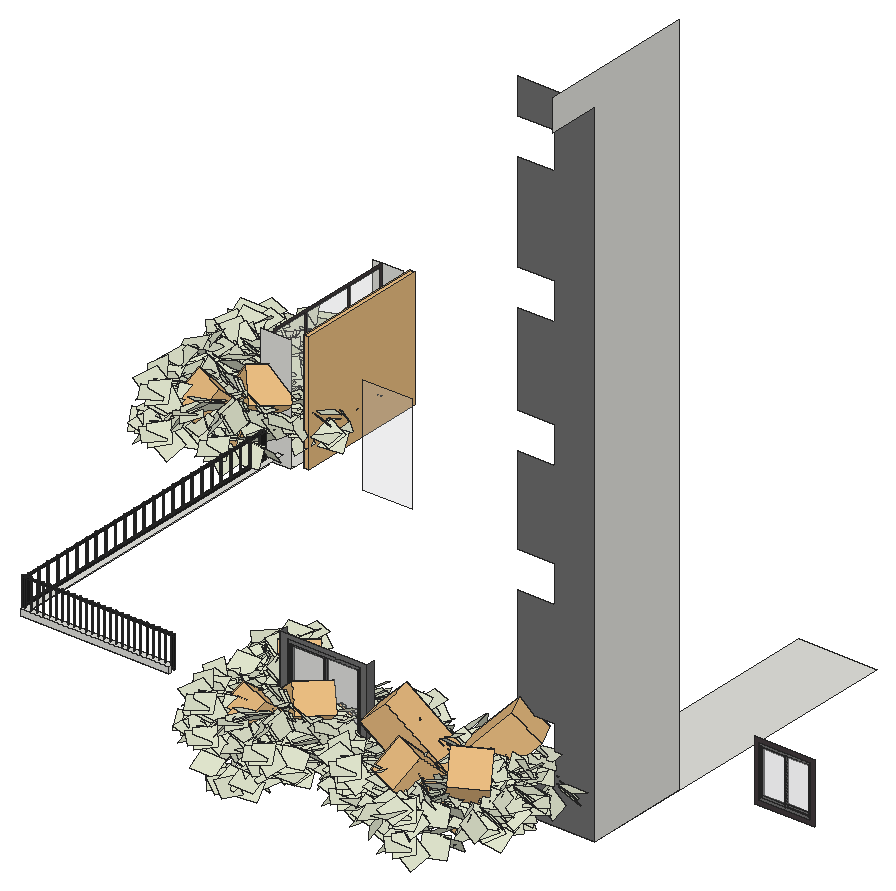
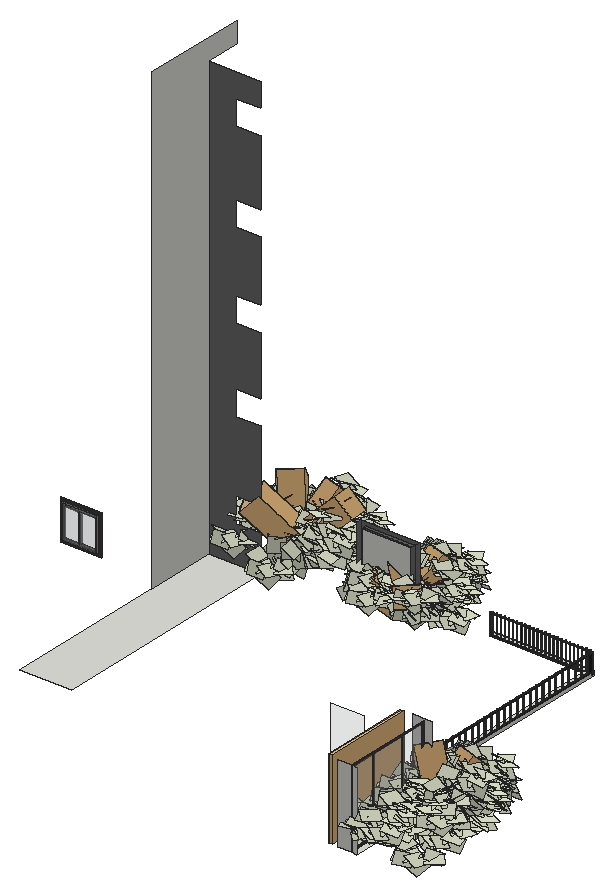
# SketchUp Ruby script. Lengths in inches.
U = 1.inch
M = Sketchup.active_model
def pt(a) = Geom::Point3d.new(a.map { |v| v * U })
def face(e, loops, mat)
  f = e.add_face(loops[0].map { |a| pt(a) })
  loops[1..].each { |l| e.add_face(l.map { |a| pt(a) }).erase! }
  f.material = f.back_material = mat if mat
  f
end
# faces: each face lists its corners as indices into pts; further lists are holes
def faces(e, pts, list, mat = nil) = list.each { |f| face(e, (f[0].is_a?(Array) ? f : [f]).map { |l| l.map { |i| pts[i] } }, mat) }
# xy, xz, yz: faces in a plane at the given z, y or x. An outline is a flat list of corners, or four numbers for a rectangle; further outlines are holes
def ring(l) = l.size == 4 ? [[l[0], l[1]], [l[2], l[1]], [l[2], l[3]], [l[0], l[3]]] : l.each_slice(2).to_a
def flat(e, list, mat, &to3) = list.each { |f| face(e, (f[0].is_a?(Array) ? f : [f]).map { |l| ring(l).map { |u, v| to3.(u, v) } }, mat) }
def xy(e, z, list, mat = nil) = flat(e, list, mat) { |x, y| [x, y, z] }
def xz(e, y, list, mat = nil) = flat(e, list, mat) { |x, z| [x, y, z] }
def yz(e, x, list, mat = nil) = flat(e, list, mat) { |y, z| [x, y, z] }
def lines(e, pts, list) = list.each { |a, b| e.add_line(pt(pts[a]), pt(pts[b])) }
# prism: a flat outline (further loops are holes) pulled along v
def prism(e, loops, v, mat = nil)
  f = face(e, loops, mat); d = Geom::Vector3d.new(v.map { |x| x * U })
  f.pushpull(f.normal.samedirection?(d) ? d.length : -d.length)
end
def box(e, o, s, mat = nil) = prism(e, [[o, [o[0] + s[0], o[1], o[2]], [o[0] + s[0], o[1] + s[1], o[2]], [o[0], o[1] + s[1], o[2]]]], [0, 0, s[2]], mat)
def at(x, y, z, deg = 0) = Geom::Transformation.translation(pt([x, y, z])) * Geom::Transformation.rotation(ORIGIN, Z_AXIS, deg.degrees)
def axes(o, x, y, z) = Geom::Transformation.new([*x, 0, *y, 0, *z, 0, *pt(o).to_a, 1])
def part(name) = M.definitions.add(name)
# library, detail: a bought-in or finely detailed component or shape, given as its bounding box
def library(name, o, s) = part(name).tap { |d| box(d.entities, o, s) }
def detail(e, o, s) = box(e.add_group.entities, o, s)
def put(e, d, t, mat = nil) = e.add_instance(d, t).tap { |i| i.material = mat if mat }
def group(e, t, mat = nil) = e.add_group.tap { |g| g.transformation = t; g.material = mat if mat }.entities
root = M.entities
M.materials.add("Celtis_australis_s cópia1").color = [224, 229, 205]
M.materials.add("Niraj_Hair_Dark").color = [109, 109, 109]
M.materials.add("[Asphalt New]").color = [67, 60, 62]
M.materials.add("[Color M08]").color = [30, 30, 30]
M.materials.add("[CoolGray4]").color = [225, 226, 230]
M.materials["[CoolGray4]"].alpha = 0.26
M.materials.add("aubin blanc").color = [238, 236, 240]
M.materials.add("bark_cherry").color = [99, 76, 62]
c1 = part("leaf1\#1")
p = [[1.6,6.78,0.04],[-9.34,-4.04,0.02],[2.67,-16.2,2.05],[13.62,-5.38,2.07]]
faces(c1.entities,p,[[0,1,2,3]],"Celtis_australis_s cópia1")
c2 = part("leaf_group1\#1")
put(c2.entities,c1,axes([-0.06,3.68,7.3125],[0.53029,-0.80282,-0.27253],[0.82812,0.42159,0.36943],[-0.18168,-0.42159,0.8884]))
put(c2.entities,c1,axes([6.4375,-3.58,5.23],[1,0,0],[0,0.98927,0.14608],[0,-0.14608,0.98927]))
put(c2.entities,c1,axes([-0.99,3.68,1.22],[0.57591,-0.80282,0.15431],[0.36532,0.42159,0.82994],[-0.73135,-0.42159,0.53609]))
put(c2.entities,c1,axes([18.71,8.59,4.39],[0.33053,0.77491,0.53877],[-0.79988,-0.073,0.5957],[0.50094,-0.62785,0.5957]))
put(c2.entities,c1,axes([13.16,0.76,0.89],[0.89618,0.3501,0.27256],[-0.44248,0.65988,0.60727],[0.03275,-0.66482,0.74628]))
put(c2.entities,c1,axes([4.53,7.98,7.3125],[-0.1927,0.94265,-0.27253],[0.88368,0.28746,0.36943],[-0.42658,0.16964,0.8884]))
put(c2.entities,c1,axes([12.46,21.28,7.16],[0.85019,0.38493,0.35918],[0.30538,-0.91629,0.25914],[-0.42887,0.11063,0.89657]))
put(c2.entities,c1,axes([6.53,15.18,2.59],[0.70711,0.70711,0],[0.5,-0.5,0.70711],[-0.5,0.5,0.70711]))
put(c2.entities,c1,axes([-3.17,8.15,3.46],[-0.03719,0.74973,0.66069],[0.94096,-0.19634,0.27576],[-0.33647,-0.63194,0.69817]))
put(c2.entities,c1,axes([23.03,17.79,4.39],[0.78166,-0.31422,0.53877],[-0.61722,-0.51398,0.5957],[-0.08973,0.79818,0.5957]))
put(c2.entities,c1,axes([14.78,21.52,3.21],[0.67246,-0.04394,0.73882],[-0.28657,-0.93583,0.20517],[-0.6824,0.3497,0.64191]))
put(c2.entities,c1,axes([10.37,-1.8125,9],[0.99279,-0.06448,-0.101],[0.11527,0.74421,0.65792],[0.03275,-0.66482,0.74628]))
put(c2.entities,c1,axes([1.45,16.1875,2.9375],[-0.2106,-0.86579,-0.45394],[0.96054,-0.26957,0.06852],[-0.18168,-0.42159,0.8884]))
c3 = library("branch1\#2",[0,0,0],[33.4,33.29,108.01])
c4 = library("fronceur+aubin+blanc+(3)",[-47.99,-0.29,1.66],[95.37,4.84,114.09])
c5 = part("branch2\#1")
p = [[13.74,0.36,0.5],[11.5,11.3125,10.98],[14.125,0.95,0],[14.97,0.95,0.19],[12.12,10.6875,11.67],[15.1,0.36,0.82],
  [11.05,10.4375,11.49],[14.34,0,1.01],[6.08,18.54,23.51],[6.83,18.32,23.89],[6.09,17.93,24.13],[3.27,29.37,34],
  [3.27,29.68,33.56],[3.73,29.59,33.82],[0,43.16,40.74],[0,43.16,40.75],[0.01,43.16,40.75],[5.59,23.2,32.77],
  [4.65,30.48,39.08],[1.92,39.79,43.02],[5.09,28.47,41.41]]
faces(c5.entities,p,[[0,1,2],[2,1,3],[3,4,5],[3,1,4],[6,0,7],[0,6,1],[5,6,7],[6,5,4],
  [6,8,1],[1,9,4],[9,1,8],[8,6,10],[4,10,6],[10,4,9],[10,11,8],[8,12,9],
  [12,8,11],[10,9,11],[13,11,9],[13,9,12],[14,12,11,15],[12,14,16,13],[13,16,15,11]],"bark_cherry")
lines(c5.entities,p,[[17,18],[11,19],[20,17],[17,10]])
c6 = part("Window sash")
g1 = group(c6.entities,at(0.98,0,0),"Niraj_Hair_Dark")
prism(g1,[[[-0.98,0,0],[30.98,0,0],[30.98,0,45.6],[-0.98,0,45.6]],[[29.01,0,43.625],[29.01,0,1.97],[0.98,0,1.97],[0.98,0,43.625]]],[0,1.18,0])
g2 = group(c6.entities,at(1.97,0.59,1.97))
xz(g2,0,[[0,0,28.03,41.66]],"[CoolGray4]")
c7 = part("Twin sash window")
put(c7.entities,c6,at(31.97,2.82,1.97))
put(c7.entities,c6,at(1.97,1.25,1.97))
g3 = group(c7.entities,at(0,0,0),"Niraj_Hair_Dark")
prism(g3,[[[65.9,4.72,0],[0,4.72,0],[0,4.72,49.53],[65.9,4.72,49.53]],[[1.97,4.72,47.5625],[1.97,4.72,1.97],[63.93,4.72,1.97],[63.93,4.72,47.5625]]],[0,-4.72,0])
c8 = part("Group\#428")
prism(c8.entities,[[[0,1.97,0],[0,1.97,1.18],[0,0,1.18],[0,0,0]],[[0,1.92,1.13],[0,1.92,0.05],[0,0.05,0.05],[0,0.05,1.13]]],[98.43,0,0])
c9 = part("Group\#430")
xy(c9.entities,0,[[0.3,0,0.22,0.01,0.15,0.04,0.09,0.09,0.04,0.15,0.01,0.22,0,0.3,0.3,0.3],[0.3,0,0.3,0.3,0.59,0.3,0.58,0.22,0.55,0.15,0.5,0.09,0.44,0.04,0.37,0.01],[0,0.3,0.01,0.37,0.04,0.44,0.09,0.5,0.15,0.55,0.22,0.58,0.3,0.59,0.3,0.3],[0.3,0.3,0.3,0.59,0.37,0.58,0.44,0.55,0.5,0.5,0.55,0.44,0.58,0.37,0.59,0.3]])
xy(c9.entities,39.37,[[0.3,0,0.37,0.01,0.44,0.04,0.5,0.09,0.55,0.15,0.58,0.22,0.59,0.3,0.58,0.37,0.55,0.44,0.5,0.5,0.44,0.55,0.37,0.58,0.3,0.59,0.22,0.58,0.15,0.55,0.09,0.5,0.04,0.44,0.01,0.37,0,0.3,0.01,0.22,0.04,0.15,0.09,0.09,0.15,0.04,0.22,0.01]])
p = [[0.09,0.09,0],[0.15,0.04,0],[0.15,0.04,39.37],[0.09,0.09,39.37],[0.22,0.01,0],[0.22,0.01,39.37],
  [0.3,0,0],[0.3,0,39.37],[0.37,0.01,0],[0.37,0.01,39.37],[0.44,0.04,0],[0.44,0.04,39.37],
  [0.5,0.09,0],[0.5,0.09,39.37],[0.01,0.22,0],[0.04,0.15,0],[0.04,0.15,39.37],[0.01,0.22,39.37],
  [0.55,0.15,0],[0.55,0.15,39.37],[0.58,0.22,0],[0.58,0.22,39.37],[0,0.3,0],[0,0.3,39.37],
  [0.59,0.3,0],[0.59,0.3,39.37],[0.01,0.37,0],[0.01,0.37,39.37],[0.58,0.37,0],[0.58,0.37,39.37],
  [0.09,0.5,0],[0.04,0.44,0],[0.04,0.44,39.37],[0.09,0.5,39.37],[0.55,0.44,0],[0.5,0.5,0],
  [0.5,0.5,39.37],[0.55,0.44,39.37],[0.15,0.55,0],[0.15,0.55,39.37],[0.44,0.55,0],[0.44,0.55,39.37],
  [0.22,0.58,0],[0.22,0.58,39.37],[0.3,0.59,0],[0.3,0.59,39.37],[0.37,0.58,0],[0.37,0.58,39.37]]
faces(c9.entities,p,[[0,1,2,3],[1,4,5,2],[4,6,7,5],[6,8,9,7],[8,10,11,9],[10,12,13,11],[14,15,16,17],[15,0,3,16],
  [12,18,19,13],[18,20,21,19],[22,14,17,23],[20,24,25,21],[26,22,23,27],[24,28,29,25],[30,31,32,33],[31,26,27,32],
  [34,35,36,37],[28,34,37,29],[38,30,33,39],[35,40,41,36],[42,38,39,43],[44,42,43,45],[46,44,45,47],[40,46,47,41]])
c10 = part("Group\#429")
prism(c10.entities,[[[0.01,0.22,35.83],[0,0.3,35.83],[0.01,0.37,35.83],[0.04,0.44,35.83],[0.09,0.5,35.83],[0.15,0.55,35.83],[0.22,0.58,35.83],[0.3,0.59,35.83],[0.37,0.58,35.83],[0.44,0.55,35.83],[0.5,0.5,35.83],[0.55,0.44,35.83],[0.58,0.37,35.83],[0.59,0.3,35.83],[0.58,0.22,35.83],[0.55,0.15,35.83],[0.5,0.09,35.83],[0.44,0.04,35.83],[0.37,0.01,35.83],[0.3,0,35.83],[0.22,0.01,35.83],[0.15,0.04,35.83],[0.09,0.09,35.83],[0.04,0.15,35.83]]],[0,0,3.54])
c11 = part("Balcony railing panel")
g4 = group(c11.entities,at(0,0,0))
put(g4,c8,axes([0,0,39.76],[1,0,0],[0,0,-1],[0,1,0]),"[Color M08]")
put(g4,c8,axes([0,0,1.97],[1,0,0],[0,0,-1],[0,1,0]),"[Color M08]")
put(g4,c8,axes([98.43,0,37.8],[0,0,-0.364],[-1,0,0],[0,1,0]),"[Color M08]")
put(g4,c8,axes([1.97,0,37.8],[0,0,-0.364],[-1,0,0],[0,1,0]),"[Color M08]")
g5 = group(c11.entities,at(1.67,0.3,1.97))
put(g5,c9,at(78.74,0,0),"[Color M08]")
put(g5,c9,at(90.55,0,0),"[Color M08]")
put(g5,c9,at(82.68,0,0),"[Color M08]")
put(g5,c9,at(86.61,0,0),"[Color M08]")
put(g5,c9,at(66.93,0,0),"[Color M08]")
put(g5,c9,at(11.8125,0,0),"[Color M08]")
put(g5,c9,at(15.75,0,0),"[Color M08]")
put(g5,c9,at(47.24,0,0),"[Color M08]")
put(g5,c9,at(59.06,0,0),"[Color M08]")
put(g5,c10,at(0,0,0),"[Color M08]")
put(g5,c9,at(39.37,0,0),"[Color M08]")
put(g5,c9,at(62.99,0,0),"[Color M08]")
put(g5,c9,at(55.12,0,0),"[Color M08]")
put(g5,c9,at(19.69,0,0),"[Color M08]")
put(g5,c9,at(35.43,0,0),"[Color M08]")
put(g5,c9,at(7.875,0,0),"[Color M08]")
put(g5,c9,at(23.62,0,0),"[Color M08]")
put(g5,c9,at(31.5,0,0),"[Color M08]")
put(g5,c9,at(43.31,0,0),"[Color M08]")
put(g5,c9,at(27.56,0,0),"[Color M08]")
put(g5,c9,at(3.9375,0,0),"[Color M08]")
put(g5,c9,at(51.18,0,0),"[Color M08]")
put(g5,c9,at(70.87,0,0),"[Color M08]")
put(g5,c9,at(74.8,0,0),"[Color M08]")
put(g5,c10,at(94.49,0,0),"[Color M08]")
xy(root,124.25,[[834.53,113.9375,888.71,360.375]])
xy(root,125.43,[[479.54,333.01,500.29,333.01,500.29,336.16,485.73,336.16,485.73,430.89,479.54,430.89],[485.73,336.16,500.29,354.38],[485.73,354.38,500.29,430.89]])
xy(root,137.74,[[944.67,187.625,980.63,190.375]],"[CoolGray4]")
xy(root,138.27,[[500.86,95.3125,500.86,311.625,502.29,311.625,502.29,96.6875,605.23,96.6875,605.23,95.3125]])
xy(root,142.68,[[500.86,95.3125,605.23,95.3125,605.23,99.4375,505.92,99.4375,505.92,319.0625,502.29,319.0625,502.29,311.625,500.86,311.625]])
xy(root,143.64,[[686.21,91.1875,747.21,96.6875]],"Niraj_Hair_Dark")
xy(root,147.57,[[691.32,91.1875,742.03,96.6875]])
xz(root,91.1875,[[686.21,143.64,686.26,195.52],[[686.26,143.64,747.21,195.52],[691.32,147.57,742.03,191.59]]],"Niraj_Hair_Dark")
xz(root,95.3125,[[500.86,138.27,605.23,142.68]])
xz(root,96.6875,[[691.32,147.57,742.03,191.59]])
xz(root,113.9375,[[834.53,124.25,888.71,124.25,888.71,585.8125,834.53,585.8125,834.53,561.09,860.28,561.09,860.28,535.34,834.53,535.34,834.53,466.13,860.28,466.13,860.28,440.38,834.53,440.38,834.53,376.25,860.28,376.25,860.28,350.5,834.53,350.5,834.53,288.82,860.28,288.82,860.28,263.07,834.53,263.07,834.53,188.57,860.28,188.57,860.28,162.82,834.53,162.82]],"Niraj_Hair_Dark")
xz(root,187.625,[[[941.43,134.5,983.87,176.94],[944.67,137.74,980.63,173.7]]],"[Asphalt New]")
xz(root,190.375,[[944.67,137.74,980.63,173.7]],"[CoolGray4]")
xz(root,311.625,[[500.86,138.27,502.29,142.68]])
xz(root,333.01,[[479.54,125.43,500.29,207.01]])
xz(root,341.53,[[543.67,123.55,578.8,193.32]],"[CoolGray4]")
xz(root,430.89,[[479.54,125.43,485.73,207.01],[485.73,125.43,500.29,207.01]])
yz(root,485.73,[[[336.16,125.43,430.89,207.01],[338.17,127.45,428.87,205]],[363.78,127.45,365.5,205],[401.16,127.45,402.66,205]],"[Asphalt New]")
yz(root,485.73,[[338.17,127.45,363.78,205],[365.5,127.45,401.16,205],[402.66,127.45,428.87,205]],"[CoolGray4]")
yz(root,500.86,[[95.3125,138.27,311.625,142.68]])
yz(root,605.23,[[95.3125,138.27,96.6875,142.68]])
yz(root,686.21,[[91.1875,143.64,96.6875,195.52]],"Niraj_Hair_Dark")
yz(root,691.32,[[91.1875,147.57,96.6875,191.59]],"Niraj_Hair_Dark")
yz(root,742.03,[[91.1875,147.57,96.6875,191.59]],"Niraj_Hair_Dark")
yz(root,747.21,[[91.1875,143.64,96.6875,195.52]],"Niraj_Hair_Dark")
yz(root,888.71,[[113.9375,124.25,187.625,124.25,187.625,607.875,76.75,607.875,76.75,604.78,77.375,604.78,77.375,590.04,76.75,590.04,76.75,585.8125,113.9375,585.8125]])
yz(root,944.67,[[187.625,137.74,190.375,173.7]],"[CoolGray4]")
yz(root,980.63,[[187.625,137.74,190.375,173.7]],"[CoolGray4]")
put(root,c2,axes([701.41,79.85,136.23],[-0.03841,-0.87984,-0.09956],[0.88915,-0.03882,0],[-0.0056,-0.12835,0.68247]))
put(root,c2,axes([733.58,84.34,136.4],[-0.03841,-0.87984,-0.09956],[0.88915,-0.03882,0],[-0.0056,-0.12835,0.68247]))
put(root,c2,axes([800.64,92.95,146.13],[0.74921,0.45418,0.15655],[-0.41604,0.75843,-0.20928],[-0.24021,0.10299,0.85076]))
put(root,c2,axes([685.95,45.36,136.88],[0.53001,-0.70334,-0.09956],[0.71079,0.53562,0],[0.07732,-0.10261,0.68247]))
put(root,c3,axes([703.43,104.55,123.28],[0.32897,-0.62866,0.04593],[-0.46078,-0.1933,0.39305],[0.25156,0.15889,0.22403]))
put(root,c2,axes([820.7,23,140.99],[0.88068,0,-0.12848],[0,0.89,0],[0.12848,0,0.88068]))
put(root,c2,axes([643.09,94.85,137.47],[0.53001,-0.70334,-0.09956],[0.71079,0.53562,0],[0.07732,-0.10261,0.68247]))
put(root,c2,axes([732.14,76.8,137.75],[0.03841,0.87984,-0.09956],[-0.88915,0.03882,0],[0.0056,0.12835,0.68247]))
put(root,c2,axes([742.58,98.3,138],[-0.7444,0.47059,-0.09956],[-0.47557,-0.75228,0],[-0.1086,0.06865,0.68247]))
put(root,c2,axes([433.31,377.82,171.25],[0.33028,-0.70334,-0.43397],[0.5516,0.53562,-0.44828],[0.61543,-0.10261,0.63468]))
put(root,c2,axes([502.43,342.86,142.75],[0.53183,0.70196,-0.12848],[-0.70939,0.53746,0],[0.07759,0.10241,0.88068]))
put(root,c2,axes([660.23,82.34,139],[0.53023,-0.70334,-0.09885],[0.71078,0.53562,0.00096],[0.07578,-0.10261,0.68258]))
put(root,c2,axes([469.24,372.3,138.98],[0.59551,-0.79027,-0.09672],[-0.79864,-0.60182,0],[0.08688,-0.11529,0.66298]))
put(root,c2,axes([472.74,372.3,138.98],[0.59551,-0.79027,-0.09672],[-0.79864,-0.60182,0],[0.08688,-0.11529,0.66298]))
put(root,c2,axes([751.33,66.63,143.55],[0.55423,-0.68442,-0.12848],[0.69166,0.5601,0],[0.08085,-0.09985,0.88068]))
put(root,c2,axes([766.63,42.29,143.55],[0.88068,0,-0.12848],[0,0.89,0],[0.12848,0,0.88068]))
put(root,c2,axes([417.23,342.88,139.36],[0.97051,-0.19308,-0.09672],[0.19512,0.98078,0],[0.14158,-0.02817,0.66298]))
put(root,c4,axes([505.98,383.9,125.11],[0,-0.97493,0],[0.73,0,0],[0,0,0.73]))
put(root,c2,axes([429.57,377.21,146.65],[-0.04359,-0.87249,0.17019],[0.84765,0.01053,0.27108],[-0.26776,0.17537,0.83045]))
put(root,c2,axes([717.63,23.22,139.68],[-0.41131,0.78137,0.08622],[-0.78924,-0.4063,-0.04978],[-0.0056,-0.12835,0.68247]))
put(root,c2,axes([672.83,114.66,142.36],[-0.04359,-0.87249,0.13189],[0.84765,0.01053,0.21007],[-0.26776,0.17537,0.64355]))
put(root,c2,axes([415.14,431.63,140.24],[-0.04316,-0.98858,-0.09672],[0.99905,-0.04362,0],[-0.0063,-0.14422,0.66298]))
put(root,c2,axes([798.51,29,150.36],[0.53001,-0.69763,0.15655],[0.71079,0.49304,-0.20928],[0.07732,0.24966,0.85076]))
put(root,c2,axes([419.74,319.6875,144.96],[0.88068,0,-0.12848],[0,0.89,0],[0.12848,0,0.88068]))
put(root,c2,axes([448.06,317.36,144.96],[-0.88068,0,-0.12848],[0,-0.89,0],[-0.12848,0,0.88068]))
put(root,c2,axes([721.99,38.76,141.06],[0.53183,0.70196,-0.09956],[-0.70939,0.53746,0],[0.07759,0.10241,0.68247]))
put(root,c2,axes([475.24,380.77,145.14],[-0.03841,-0.87984,-0.12848],[0.88915,-0.03882,0],[-0.0056,-0.12835,0.88068]))
put(root,c2,axes([467.64,352.46,144.43],[-0.41131,0.78137,0.11126],[-0.78924,-0.4063,-0.06424],[-0.0056,-0.12835,0.88068]))
put(root,c2,axes([804.11,139.8,145.35],[-0.03841,-0.87984,-0.12848],[0.88915,-0.03882,0],[-0.0056,-0.12835,0.88068]))
put(root,c2,axes([677.34,100.59,142.3],[0.03764,0.88184,0.0885],[-0.86164,0.00793,0.17262],[0.21969,-0.11998,0.66186]))
put(root,c2,axes([699.91,40.99,146.36],[0.74921,0.45418,0.12132],[-0.41604,0.75843,-0.16218],[-0.24021,0.10299,0.65929]))
put(root,c2,axes([414.45,387.5625,141.6],[0.59576,-0.79027,-0.09602],[0.79863,0.60182,0.00093],[0.08515,-0.11529,0.66308]))
put(root,c2,axes([435.66,289.74,146.22],[0.88059,0.0123,-0.12848],[-0.01243,0.88991,0],[0.12846,0.00179,0.88068]))
put(root,c3,axes([472.91,323.63,128.74],[-0.66136,0.25698,0.05927],[0.21982,0.44874,0.50721],[-0.0849,-0.28517,0.28909]))
put(root,c2,axes([465.25,397.4375,142.5],[0.59551,-0.79027,-0.09672],[0.79864,0.60182,0],[0.08688,-0.11529,0.66298]))
put(root,c3,axes([452.4375,401.37,129.38],[0.48871,-0.35814,0.03391],[-0.28049,-0.32155,0.29019],[0.17031,0.27706,0.21171]))
put(root,c2,axes([429.61,358.75,142.75],[0.93562,-0.32216,-0.09672],[0.32557,0.94552,0],[0.13649,-0.047,0.66298]))
put(root,c3,axes([701.49,105.65,129.7],[-0.52875,-0.46238,0.02425],[0.31975,-0.32962,0.41258],[-0.2583,0.31925,0.27339]))
put(root,c3,axes([829.23,65.52,129.82],[-0.66136,0.25698,0.05927],[0.21982,0.44874,0.50721],[-0.10884,-0.3656,0.37063]))
put(root,c5,axes([452.16,396.1,139.43],[0.29715,-0.71035,0],[-0.64116,-0.2682,-0.2221],[-0.21713,-0.09083,0.33061]))
put(root,c2,axes([447.94,412.25,143.59],[0.59551,-0.79027,-0.09672],[0.79864,0.60182,0],[0.08688,-0.11529,0.66298]))
put(root,c2,axes([863.93,63.18,148.52],[-0.04763,0.87939,-0.12848],[-0.8887,-0.04813,0],[-0.00695,0.12829,0.88068]))
put(root,c2,axes([852.2,48.96,148.52],[0.75804,0.4483,-0.12848],[-0.45305,0.76606,0],[0.11059,0.0654,0.88068]))
put(root,c2,axes([853.78,123.73,149.52],[-0.03841,-0.87984,-0.12848],[0.88915,-0.03882,0],[-0.0056,-0.12835,0.88068]))
put(root,c2,axes([475.91,353.9,149.58],[0.86375,-0.17184,-0.12848],[0.17366,0.87289,0],[0.12601,-0.02507,0.88068]))
put(root,c2,axes([475.91,293.66,149.58],[0.86375,-0.17184,-0.12848],[0.17366,0.87289,0],[0.12601,-0.02507,0.88068]))
put(root,c2,axes([666.67,126,168.4],[0.33028,-0.70334,-0.3363],[0.5516,0.53562,-0.34739],[0.61543,-0.10261,0.49184]))
put(root,c2,axes([452.32,387.4375,145.89],[0.59551,-0.79027,-0.09672],[0.79864,0.60182,0],[0.08688,-0.11529,0.66298]))
put(root,c2,axes([465.25,377.625,145.89],[0.59551,-0.79027,-0.09672],[0.79864,0.60182,0],[0.08688,-0.11529,0.66298]))
put(root,c2,axes([469.24,372.3,145.89],[0.59551,-0.79027,-0.09672],[-0.79864,-0.60182,0],[0.08688,-0.11529,0.66298]))
put(root,c2,axes([735.79,91.05,146.32],[0.53183,0.70196,-0.09956],[-0.70939,0.53746,0],[0.07759,0.10241,0.68247]))
put(root,c2,axes([459.19,420.75,146.27],[0.59551,-0.79027,-0.09672],[0.79864,0.60182,0],[0.08688,-0.11529,0.66298]))
put(root,c2,axes([766.63,47.01,150.84],[0.88068,0,-0.12848],[0,0.89,0],[0.12848,0,0.88068]))
put(root,c2,axes([662.93,125.4,149.34],[-0.04359,-0.87249,0.13189],[0.84765,0.01053,0.21007],[-0.26776,0.17537,0.64355]))
put(root,c2,axes([454.25,297.3,157.61],[0.87255,-0.07903,0.15655],[0.1152,0.85734,-0.20928],[-0.13223,0.22544,0.85076]))
put(root,c2,axes([653.1,67.875,148.03],[0.88068,0,-0.09956],[0,0.89,0],[0.12848,0,0.68247]))
put(root,c2,axes([681.42,65.55,148.03],[-0.88068,0,-0.09956],[0,-0.89,0],[-0.12848,0,0.68247]))
put(root,c2,axes([708.6,128.95,148.17],[-0.03841,-0.87984,-0.09956],[0.88915,-0.03882,0],[-0.0056,-0.12835,0.68247]))
put(root,c2,axes([701,100.65,147.61],[-0.41131,0.78137,0.08622],[-0.78924,-0.4063,-0.04978],[-0.0056,-0.12835,0.68247]))
put(root,c2,axes([781.48,83.74,152.4],[0.7444,0.47059,-0.12848],[-0.47557,0.75228,0],[0.1086,0.06865,0.88068]))
put(root,c2,axes([423.8,387.5625,169.79],[0.3711,-0.79027,-0.32669],[0.61978,0.60182,-0.33747],[0.69149,-0.11529,0.4778]))
put(root,c2,axes([669.02,37.93,149],[0.88059,0.0123,-0.09956],[-0.01243,0.88991,0],[0.12846,0.00179,0.68247]))
put(root,c3,axes([706.27,71.82,135.45],[-0.66136,0.25698,0.04593],[0.21982,0.44874,0.39305],[-0.0849,-0.28517,0.22403]))
put(root,c2,axes([486.84,363.8,153.19],[-0.03841,-0.87984,-0.12848],[0.88915,-0.03882,0],[-0.0056,-0.12835,0.88068]))
put(root,c2,axes([798.51,51.9375,158.23],[0.53001,-0.68244,-0.21324],[0.71079,0.53162,0.06528],[0.07732,-0.20917,0.86161]))
put(root,c2,axes([820.06,10.46,159.31],[0.74921,0.45418,0.15655],[-0.41604,0.75843,-0.20928],[-0.24021,0.10299,0.85076]))
put(root,c3,axes([839.09,81.78,136.1],[-0.57341,-0.41789,0.05927],[-0.259,0.42733,0.50721],[0.24895,-0.28903,0.37063]))
put(root,c2,axes([800.64,92.95,159.87],[0.74921,0.45418,0.15655],[-0.41604,0.75843,-0.20928],[-0.24021,0.10299,0.85076]))
put(root,c2,axes([419.74,326.97,154.53],[0.88068,0,-0.12848],[0,0.89,0],[0.12848,0,0.88068]))
put(root,c2,axes([484.4,332.46,154.6],[0.53183,0.70196,-0.12848],[-0.70939,0.53746,0],[0.07759,0.10241,0.88068]))
put(root,c3,axes([465.4375,360.54,153.88],[-0.4587,-0.54131,0.05927],[0.35246,-0.35421,-0.50721],[0.24186,-0.1733,0.28909]))
put(root,c2,axes([485.8,344.91,154.7],[-0.4192,-0.77451,-0.12848],[0.78271,-0.42363,0],[-0.06115,-0.11299,0.88068]))
put(root,c5,axes([445.41,383.35,147.01],[0.74841,0.18106,0],[0.16342,-0.6755,-0.2221],[0.07795,-0.3222,0.46564]))
put(root,c7,axes([944.67,187.625,137.74],[0.54567,0,0],[0,0.58158,0],[0,0,0.72599]))
put(root,c2,axes([709.27,102.09,151.61],[0.86375,-0.17184,-0.09956],[0.17366,0.87289,0],[0.12601,-0.02507,0.68247]))
put(root,c2,axes([709.27,41.85,151.61],[0.86375,-0.17184,-0.09956],[0.17366,0.87289,0],[0.12601,-0.02507,0.68247]))
put(root,c2,axes([447.67,364.48,155.23],[-0.41131,0.78137,0.11126],[-0.78924,-0.4063,-0.06424],[-0.0056,-0.12835,0.88068]))
put(root,c2,axes([447.67,352.46,155.23],[-0.41131,0.78137,0.11126],[-0.78924,-0.4063,-0.06424],[-0.0056,-0.12835,0.88068]))
put(root,c2,axes([784.43,82.34,185.21],[0.33028,-0.70334,-0.43397],[0.5516,0.53562,-0.44828],[0.61543,-0.10261,0.63468]))
put(root,c2,axes([443,308.34,156.75],[0.53001,-0.70334,-0.12848],[0.71079,0.53562,0],[0.07732,-0.10261,0.88068]))
put(root,c2,axes([687.61,45.49,157.83],[0.87255,-0.07903,0.12132],[0.1152,0.85734,-0.16218],[-0.13223,0.22544,0.65929]))
put(root,c2,axes([768.91,83.74,157.4],[0.7444,0.47059,-0.12848],[-0.47557,0.75228,0],[0.1086,0.06865,0.88068]))
put(root,c2,axes([846.11,65.375,157.53],[-0.03841,-0.87984,-0.12848],[0.88915,-0.03882,0],[-0.0056,-0.12835,0.88068]))
put(root,c11,axes([500.29,97.6875,140.125],[1.07895,0,0],[0,0.5551,0],[0,0,0.5551]),"aubin blanc")
put(root,c2,axes([447.94,426.125,153.89],[0.59551,-0.79027,-0.09672],[0.79864,0.60182,0],[0.08688,-0.11529,0.66298]))
put(root,c2,axes([720.2,111.99,154.41],[-0.03841,-0.87984,-0.09956],[0.88915,-0.03882,0],[-0.0056,-0.12835,0.68247]))
put(root,c2,axes([459.57,412.25,154.89],[0.59551,-0.79027,-0.09672],[0.79864,0.60182,0],[0.08688,-0.11529,0.66298]))
put(root,c2,axes([798.51,49.58,165.16],[0.53001,-0.69763,0.15655],[0.71079,0.49304,-0.20928],[0.07732,0.24966,0.85076]))
put(root,c2,axes([653.1,75.16,155.44],[0.88068,0,-0.09956],[0,0.89,0],[0.12848,0,0.68247]))
put(root,c2,axes([871.05,66.39,159.42],[0.03841,0.87984,-0.12848],[-0.88915,0.03882,0],[0.0056,0.12835,0.88068]))
put(root,c2,axes([442.95,354.4375,155.08],[0.59576,-0.79027,-0.09602],[0.79863,0.60182,0.00093],[0.08515,-0.11529,0.66308]))
put(root,c2,axes([717.76,80.65,155.5],[0.53183,0.70196,-0.09956],[-0.70939,0.53746,0],[0.07759,0.10241,0.68247]))
put(root,c3,axes([698.8,108.73,154.9375],[-0.4587,-0.54131,0.04593],[0.35246,-0.35421,-0.39305],[0.24186,-0.1733,0.22403]))
put(root,c2,axes([719.16,93.1,155.57],[-0.4192,-0.77451,-0.09956],[0.78271,-0.42363,0],[-0.06115,-0.11299,0.68247]))
put(root,c3,axes([809.48,67.59,142.39],[-0.12279,0.69882,0.05927],[0.49771,0.04443,0.50721],[-0.36911,-0.09629,0.37063]))
put(root,c11,axes([501.875,98.3125,142.83],[0,2.13828,0],[-1.34885,0,0],[0,0,0.45928]),"aubin blanc")
put(root,c2,axes([681.03,112.67,155.98],[-0.41131,0.78137,0.08622],[-0.78924,-0.4063,-0.04978],[-0.0056,-0.12835,0.68247]))
put(root,c2,axes([681.03,100.65,155.98],[-0.41131,0.78137,0.08622],[-0.78924,-0.4063,-0.04978],[-0.0056,-0.12835,0.68247]))
put(root,c2,axes([820.7,23,160.96],[0.88068,0,-0.12848],[0,0.89,0],[0.12848,0,0.88068]))
put(root,c2,axes([766.63,42.29,160.96],[0.88068,0,-0.12848],[0,0.89,0],[0.12848,0,0.88068]))
put(root,c2,axes([676.36,56.53,157.17],[0.53001,-0.70334,-0.09956],[0.71079,0.53562,0],[0.07732,-0.10261,0.68247]))
put(root,c2,axes([422.35,393.37,157.6],[0.18564,-0.97211,-0.09602],[0.98229,0.18738,0.00093],[0.0255,-0.14104,0.66308]))
put(root,c2,axes([448.4,344.85,159.5625],[0.9012,0.40902,-0.09602],[-0.4131,0.91068,0.00093],[0.13109,0.05795,0.66308]))
put(root,c2,axes([448.24,405.76,160.25],[0.94927,-0.27938,-0.09672],[0.28234,0.95931,0],[0.13848,-0.04076,0.66298]))
put(root,c5,axes([453.26,395.04,149.35],[0.22289,-0.71035,-0.13166],[-0.70016,-0.2682,0.11748],[0.16345,-0.09083,0.3442]))
put(root,c7,axes([691.32,91.1875,147.57],[0.7693,0,0],[0,0.7553,0],[0,0,0.89881]))
put(root,c2,axes([475.63,326.85,165.27],[0.53001,-0.70334,-0.12848],[-0.71079,-0.53562,0],[0.07732,-0.10261,0.88068]))
put(root,c2,axes([478.75,326.85,165.27],[0.53001,-0.70334,-0.12848],[-0.71079,-0.53562,0],[0.07732,-0.10261,0.88068]))
put(root,c2,axes([821.56,79.85,165.43],[-0.03841,-0.87984,-0.12848],[0.88915,-0.03882,0],[-0.0056,-0.12835,0.88068]))
put(root,c2,axes([853.73,84.34,165.65],[-0.03841,-0.87984,-0.12848],[0.88915,-0.03882,0],[-0.0056,-0.12835,0.88068]))
put(root,c2,axes([429.35,300.67,165.77],[0.86375,-0.17184,-0.12848],[0.17366,0.87289,0],[0.12601,-0.02507,0.88068]))
put(root,c2,axes([806.1,45.36,166.27],[0.53001,-0.70334,-0.12848],[0.71079,0.53562,0],[0.07732,-0.10261,0.88068]))
put(root,c3,axes([823.58,104.55,148.72],[0.32897,-0.62866,0.05927],[-0.46078,-0.1933,0.50721],[0.25156,0.15889,0.28909]))
put(root,c2,axes([459.88,368.49,162.5],[0.98574,0.08818,-0.09602],[-0.08889,0.99604,0.00093],[0.14287,0.01137,0.66308]))
put(root,c2,axes([427.49,379.65,166.93],[-0.03841,-0.87984,-0.12848],[0.88915,-0.03882,0],[-0.0056,-0.12835,0.88068]))
put(root,c2,axes([763.24,94.85,167.03],[0.53001,-0.70334,-0.12848],[0.71079,0.53562,0],[0.07732,-0.10261,0.88068]))
put(root,c2,axes([852.29,76.8,167.39],[0.03841,0.87984,-0.12848],[-0.88915,0.03882,0],[0.0056,0.12835,0.88068]))
put(root,c2,axes([862.73,98.3,167.71],[-0.7444,0.47059,-0.12848],[-0.47557,-0.75228,0],[-0.1086,0.06865,0.88068]))
put(root,c2,axes([708.99,75.04,163.76],[0.53001,-0.70334,-0.09956],[-0.71079,-0.53562,0],[0.07732,-0.10261,0.68247]))
put(root,c2,axes([712.11,75.04,163.76],[0.53001,-0.70334,-0.09956],[-0.71079,-0.53562,0],[0.07732,-0.10261,0.68247]))
put(root,c2,axes([662.71,48.86,164.15],[0.86375,-0.17184,-0.09956],[0.17366,0.87289,0],[0.12601,-0.02507,0.68247]))
put(root,c2,axes([426.87,340.4375,168.75],[0.53023,-0.70334,-0.12755],[0.71078,0.53562,0.00124],[0.07578,-0.10261,0.88081]))
put(root,c2,axes([780.38,82.34,169.01],[0.53023,-0.70334,-0.12755],[0.71078,0.53562,0.00124],[0.07578,-0.10261,0.88081]))
put(root,c2,axes([660.85,127.84,165.06],[-0.03841,-0.87984,-0.09956],[0.88915,-0.03882,0],[-0.0056,-0.12835,0.68247]))
put(root,c5,axes([466.03,382.64,154.21],[-0.59925,-0.02343,-0.16233],[-0.03641,0.39798,0.03456],[-0.19849,-0.08282,0.33428]))
